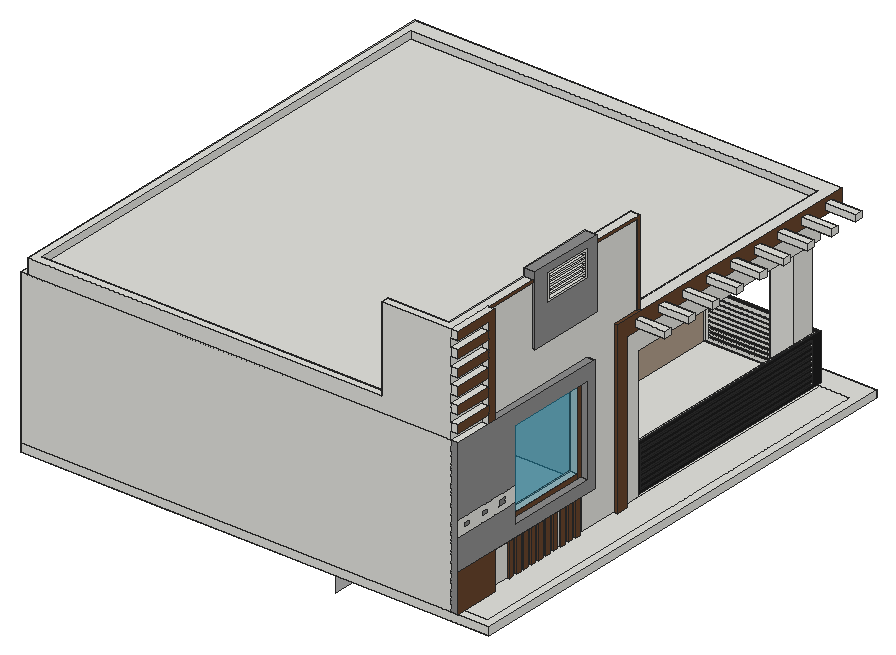
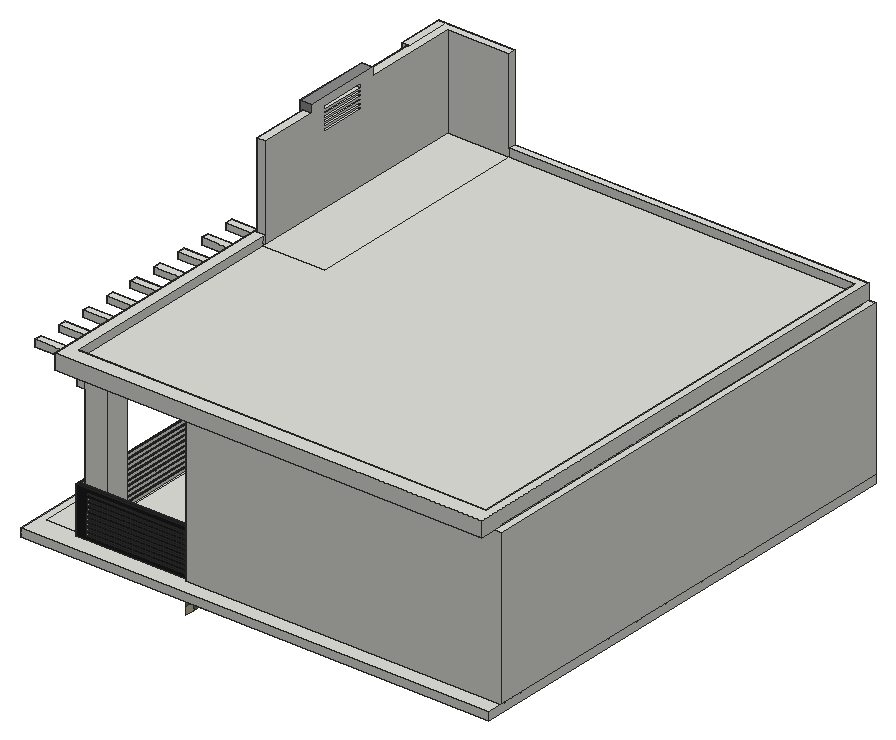
# SketchUp Ruby script. Lengths in inches.
U = 1.inch
M = Sketchup.active_model
def pt(a) = Geom::Point3d.new(a.map { |v| v * U })
def face(e, loops, mat)
  f = e.add_face(loops[0].map { |a| pt(a) })
  loops[1..].each { |l| e.add_face(l.map { |a| pt(a) }).erase! }
  f.material = f.back_material = mat if mat
  f
end
# faces: each face lists its corners as indices into pts; further lists are holes
def faces(e, pts, list, mat = nil) = list.each { |f| face(e, (f[0].is_a?(Array) ? f : [f]).map { |l| l.map { |i| pts[i] } }, mat) }
# xy, xz, yz: faces in a plane at the given z, y or x. An outline is a flat list of corners, or four numbers for a rectangle; further outlines are holes
def ring(l) = l.size == 4 ? [[l[0], l[1]], [l[2], l[1]], [l[2], l[3]], [l[0], l[3]]] : l.each_slice(2).to_a
def flat(e, list, mat, &to3) = list.each { |f| face(e, (f[0].is_a?(Array) ? f : [f]).map { |l| ring(l).map { |u, v| to3.(u, v) } }, mat) }
def xy(e, z, list, mat = nil) = flat(e, list, mat) { |x, y| [x, y, z] }
def xz(e, y, list, mat = nil) = flat(e, list, mat) { |x, z| [x, y, z] }
def yz(e, x, list, mat = nil) = flat(e, list, mat) { |y, z| [x, y, z] }
def lines(e, pts, list) = list.each { |a, b| e.add_line(pt(pts[a]), pt(pts[b])) }
# prism: a flat outline (further loops are holes) pulled along v
def prism(e, loops, v, mat = nil)
  f = face(e, loops, mat); d = Geom::Vector3d.new(v.map { |x| x * U })
  f.pushpull(f.normal.samedirection?(d) ? d.length : -d.length)
end
def box(e, o, s, mat = nil) = prism(e, [[o, [o[0] + s[0], o[1], o[2]], [o[0] + s[0], o[1] + s[1], o[2]], [o[0], o[1] + s[1], o[2]]]], [0, 0, s[2]], mat)
def at(x, y, z, deg = 0) = Geom::Transformation.translation(pt([x, y, z])) * Geom::Transformation.rotation(ORIGIN, Z_AXIS, deg.degrees)
def axes(o, x, y, z) = Geom::Transformation.new([*x, 0, *y, 0, *z, 0, *pt(o).to_a, 1])
def part(name) = M.definitions.add(name)
# library, detail: a bought-in or finely detailed component or shape, given as its bounding box
def library(name, o, s) = part(name).tap { |d| box(d.entities, o, s) }
def detail(e, o, s) = box(e.add_group.entities, o, s)
def put(e, d, t, mat = nil) = e.add_instance(d, t).tap { |i| i.material = mat if mat }
def group(e, t, mat = nil) = e.add_group.tap { |g| g.transformation = t; g.material = mat if mat }.entities
root = M.entities
M.materials.add("Brick_01_1K").color = [147, 115, 98]
M.materials.add("Brick_05_1K").color = [195, 185, 161]
M.materials.add("Brick_20_1K1").color = [126, 109, 93]
M.materials.add("Glass_Basic_01").color = [33, 150, 186]
M.materials["Glass_Basic_01"].alpha = 0.4
M.materials.add("M02_Ash_Whisper").color = [196, 196, 196]
M.materials.add("M04_Stone_Frost").color = [142, 142, 142]
M.materials.add("M08_Obsidian_Black").color = [30, 30, 30]
M.materials.add("ThomThom - Complexion2").color = [175, 156, 137]
M.materials.add("ThomThom - Waistcoat2").color = [127, 127, 126]
M.materials.add("Wood_Veneer_15_1K").color = [103, 69, 45]
xy(root,144,[[57,57,174,66],[174,57,180,66],[180,57,294,66],[294,57,303,423],[[303,57,423,435],[309,63,417,429]],
  [[309,63,309,429,417,429,417,81,405,81,405,63],[369,399,387,417]],[57,66,66,423],[66,66,174,234],[174,66,180,414],[180,66,294,234],
  [66,234,174,240],[180,234,294,240],[66,240,174,414],[180,240,294,414],[66,414,174,423],
  [174,414,180,423],[180,414,294,423],[57,423,66,435],[66,423,174,435],[174,423,180,435],
  [180,423,294,435],[294,423,303,435]])
xy(root,150,[[399,57,423,57,423,435,57,435,57,423,303,423,303,420.78,391,420.78,391,417,417,417,417,63,399,63],[63,63,174,234],[180,63,387,234],[399,63,417,63,417,417,393,417,393,225,396,225,396,216,393,216,393,180.2,395,180.2,395,176.6,393,176.6,393,173,395,173,395,169.4,393,169.4,393,165.8,395,165.8,395,162.2,393,162.2,393,158.6,395,158.6,395,155,393,155,393,151.4,395,151.4,395,147.8,393,147.8,393,144.2,395,144.2,395,140.6,393,140.6,393,137,395,137,395,133.4,393,133.4,393,129.8,395,129.8,395,126.2,393,126.2,393,122.6,395,122.6,395,119,393,119,393,115.4,395,115.4,395,111.8,393,111.8,393,93,399,93],[63,240,174,417],
  [180,240,297,417],[303,240,387,240,387,399,369,399,369,417,303,417],[387,240,393,240,393,417,391,417,391,242,389,242,389,417,387,417],[303,417,389,417.78]])
xy(root,152,[[389,244,391,413]],"M08_Obsidian_Black")
xy(root,153,[[297,255,303,297]])
xy(root,153,[[306,417.78,382.19,420.78]],"M08_Obsidian_Black")
xy(root,153.88,[[389,244,391,413]],"M08_Obsidian_Black")
xy(root,154.76,[[306,417.78,382.19,420.78]])
xy(root,155.76,[[389,244,391,413]],"M08_Obsidian_Black")
xy(root,156.53,[[306,417.78,382.19,420.78]],"M08_Obsidian_Black")
xy(root,157.65,[[389,244,391,413]],"M08_Obsidian_Black")
xy(root,158.29,[[306,417.78,382.19,420.78]],"M08_Obsidian_Black")
xy(root,159.53,[[389,244,391,413]],"M08_Obsidian_Black")
xy(root,160.06,[[306,417.78,382.19,420.78]],"M08_Obsidian_Black")
xy(root,161.41,[[389,244,391,413]],"M08_Obsidian_Black")
xy(root,161.82,[[306,417.78,382.19,420.78]],"M08_Obsidian_Black")
xy(root,163.29,[[389,244,391,413]],"M08_Obsidian_Black")
xy(root,163.59,[[306,417.78,382.19,420.78]],"M08_Obsidian_Black")
xy(root,165.18,[[389,244,391,413]],"M08_Obsidian_Black")
xy(root,165.35,[[306,417.78,382.19,420.78]],"M08_Obsidian_Black")
xy(root,167.06,[[389,244,391,413]],"M08_Obsidian_Black")
xy(root,167.12,[[306,417.78,382.19,420.78]],"M08_Obsidian_Black")
xy(root,168.88,[[306,417.78,382.19,420.78]],"M08_Obsidian_Black")
xy(root,168.94,[[389,244,391,413]],"M08_Obsidian_Black")
xy(root,170.65,[[306,417.78,382,420.78]],"M08_Obsidian_Black")
xy(root,170.82,[[389,244,391,413]],"M08_Obsidian_Black")
xy(root,172.41,[[306,417.78,382,420.78]],"M08_Obsidian_Black")
xy(root,172.71,[[389,244,391,413]],"M08_Obsidian_Black")
xy(root,174.18,[[306,417.78,382,420.78]],"M08_Obsidian_Black")
xy(root,174.59,[[389,244,391,413]],"M08_Obsidian_Black")
xy(root,175.94,[[306,417.78,382,420.78]],"M08_Obsidian_Black")
xy(root,176.47,[[389,244,391,413]],"M08_Obsidian_Black")
xy(root,177.71,[[306,417.78,382,420.78]],"M08_Obsidian_Black")
xy(root,178.35,[[389,244,391,413]],"M08_Obsidian_Black")
xy(root,179.47,[[306,417.78,382,420.78]],"M08_Obsidian_Black")
xy(root,180,[[393,93,399,111.8],[395,111.8,395,115.4,393,115.4,393,119,395,119,395,122.6,393,122.6,393,126.2,395,126.2,395,129.8,393,129.8,393,133.4,395,133.4,395,137,393,137,393,140.6,395,140.6,395,144.2,393,144.2,393,147.8,395,147.8,395,151.4,393,151.4,393,155,395,155,395,158.6,393,158.6,393,162.2,395,162.2,395,165.8,393,165.8,393,169.4,395,169.4,395,173,393,173,393,176.6,395,176.6,395,180.2,393,180.2,393,183.8,399,183.8,399,111.8],[393,183.8,399,189.8]])
xy(root,180.24,[[389,244,391,413]],"M08_Obsidian_Black")
xy(root,181.24,[[306,417.78,382,420.78]],"M08_Obsidian_Black")
xy(root,182.12,[[389,244,391,413]],"M08_Obsidian_Black")
xy(root,183,[[306,417.78,382,420.78]],"M08_Obsidian_Black")
xy(root,184,[[389,244,391,413]],"M08_Obsidian_Black")
xy(root,186,[[389,242,391,242,391,420.78,303,420.78,303,417.78,389,417.78]],"M08_Obsidian_Black")
xy(root,189,[[297,327,303,369]])
xy(root,189,[[393,111.8,399,183.8]],"M04_Stone_Frost")
xy(root,192,[[387,114.8,393,180.8]])
xy(root,231,[[297,255,303,297],[297,327,303,369]])
xy(root,252,[[381,240,381,399,387,399,387,417,393,417,393,240]])
xy(root,255,[[387,114.8,393,180.8]])
xy(root,258,[[393,111.8,399,183.8]],"M04_Stone_Frost")
xy(root,270,[[57,57,63,423],[63,57,174,63],[174,57,180,63],[180,57,387,63],[393,57,399,87],
  [63,63,174,234],[174,63,180,417],[180,63,387,234],[393,225,396,240],[63,234,174,240],
  [180,234,387,234,387,240,303,240,303,417,297,417,297,240,180,240],[393,240,393,417,303,417,303,423,63,423,63,435,396,435,396,240],[63,240,174,417],[180,240,297,417],[303,240,303,417,369,417,369,399,381,399,381,240],
  [63,417,174,423],[174,417,180,423],[180,417,297,423],[297,417,303,423]])
xy(root,270,[[393,93,399,189.8]],"M04_Stone_Frost")
xy(root,273.58,[[396,232.62,420,238.62],[396,255.85,420,261.85],[396,279.07,420,285.07],[396,302.29,420,308.29],[396,325.52,420,331.52],
  [396,348.74,420,354.74],[396,371.97,420,377.97],[396,395.19,420,401.19],[396,418.41,420,424.41]])
xy(root,276,[[69,63,339,63,339,243,387,243,387,423,69,423],[339,63,387,243]])
xy(root,276.55,[[393,57,399,87]])
xy(root,278.58,[[396,232.62,420,238.62],[396,255.85,420,261.85],[396,279.07,420,285.07],[396,302.29,420,308.29],[396,325.52,420,331.52],
  [396,348.74,420,354.74],[396,371.97,420,377.97],[396,395.19,420,401.19],[396,418.41,420,424.41]])
xy(root,282,[[63,57,339,57,339,63,69,63,69,423,387,423,387,240,396,240,396,435,63,435]])
xy(root,282,[[393,216,396,216,396,240,394,240,394,238,393,238]],"Wood_Veneer_15_1K")
xy(root,283.09,[[393,57,399,87]])
xy(root,289.64,[[393,57,399,87]])
xy(root,296.18,[[393,57,399,87]])
xy(root,300,[[393,135.8,396,195.8]])
xy(root,302.73,[[393,57,399,87]])
xy(root,309.27,[[393,57,399,87]])
xy(root,315.82,[[393,57,399,87]])
xy(root,322.36,[[393,57,399,87]])
xy(root,328.91,[[393,57,399,87]])
xy(root,329,[[396,146.8,397,184.8]])
xy(root,330,[[387,147.8,397,183.8]])
xy(root,332,[[387,147.8,396,183.8]])
xy(root,333,[[387,147.8,396,183.8]])
xy(root,335,[[387,147.8,396,183.8]])
xy(root,335.45,[[393,57,399,87]])
xy(root,336,[[387,147.8,396,183.8]])
xy(root,338,[[387,147.8,396,183.8]])
xy(root,339,[[387,147.8,396,183.8]])
xy(root,341,[[387,147.8,396,183.8]])
xy(root,342,[[393,57,399,87],[387,147.8,396,183.8]])
xy(root,344,[[387,147.8,396,183.8]])
xy(root,345,[[387,147.8,396,183.8]])
xy(root,346,[[393,93,394,135.8],[393,195.8,394,238]])
xy(root,348,[[339,57,393,57,393,93,394,93,394,135.8,387,135.8,387,63,339,63],[393,57,399,93],[387,147.8,397,183.8],[387,195.8,394,240]])
xy(root,349,[[396,146.8,397,184.8]])
xy(root,354,[[387,135.8,396,195.8]],"M04_Stone_Frost")
xz(root,57,[[57,144,423,150],[57,150,393,270],[63,270,393,270,393,348,339,348,339,282,63,282],[393,276.55,399,283.09],[393,289.64,399,296.18],
  [393,302.73,399,309.27],[393,315.82,399,322.36],[393,328.91,399,335.45],[393,342,399,348]])
xz(root,57,[[393,150,399,270]],"M04_Stone_Frost")
xz(root,63,[[63,150,174,270],[174,150,180,270],[180,150,387,270],[69,276,339,282],[339,276,387,348]])
xz(root,87,[[393,270,399,276.55],[393,283.09,399,289.64],[393,296.18,399,302.73],[393,309.27,399,315.82],[393,322.36,399,328.91],
  [393,335.45,399,342]])
xz(root,93,[[393,270,393,346,394,346,394,348,399,348,399,270]])
xz(root,93,[[393,150,399,180]],"Wood_Veneer_15_1K")
xz(root,111.8,[[393,189,399,258]],"M04_Stone_Frost")
xz(root,111.8,[[393,150,395,180]],"Wood_Veneer_15_1K")
xz(root,114.8,[[387,192,393,255]])
xz(root,115.4,[[393,150,395,180]],"Wood_Veneer_15_1K")
xz(root,119,[[393,150,395,180]],"Wood_Veneer_15_1K")
xz(root,122.6,[[393,150,395,180]],"Wood_Veneer_15_1K")
xz(root,126.2,[[393,150,395,180]],"Wood_Veneer_15_1K")
xz(root,129.8,[[393,150,395,180]],"Wood_Veneer_15_1K")
xz(root,133.4,[[393,150,395,180]],"Wood_Veneer_15_1K")
xz(root,135.8,[[393,300,396,300,396,354,387,354,387,348,394,348,394,346,393,346]],"M04_Stone_Frost")
xz(root,137,[[393,150,395,180]],"Wood_Veneer_15_1K")
xz(root,140.6,[[393,150,395,180]],"Wood_Veneer_15_1K")
xz(root,144.2,[[393,150,395,180]],"Wood_Veneer_15_1K")
xz(root,146.8,[[396,329,397,349]])
xz(root,147.8,[[387,330,397,332],[396,332,397,333],[387,333,397,335],[396,335,397,336],[387,336,397,338],
  [396,338,397,339],[387,339,397,341],[396,341,397,342],[387,342,397,344],[396,344,397,345],
  [387,345,397,348]])
xz(root,147.8,[[393,150,395,180]],"Wood_Veneer_15_1K")
xz(root,151.4,[[393,150,395,180]],"Wood_Veneer_15_1K")
xz(root,155,[[393,150,395,180]],"Wood_Veneer_15_1K")
xz(root,158.6,[[393,150,395,180]],"Wood_Veneer_15_1K")
xz(root,162.2,[[393,150,395,180]],"Wood_Veneer_15_1K")
xz(root,165.8,[[393,150,395,180]],"Wood_Veneer_15_1K")
xz(root,169.4,[[393,150,395,180]],"Wood_Veneer_15_1K")
xz(root,173,[[393,150,395,180]],"Wood_Veneer_15_1K")
xz(root,176.6,[[393,150,395,180]],"Wood_Veneer_15_1K")
xz(root,180.2,[[393,150,395,180]],"Wood_Veneer_15_1K")
xz(root,180.8,[[387,192,393,255]])
xz(root,183.8,[[387,330,397,332],[396,332,397,333],[387,333,397,335],[396,335,397,336],[387,336,397,338],
  [396,338,397,339],[387,339,397,341],[396,341,397,342],[387,342,397,344],[396,344,397,345],
  [387,345,397,348]])
xz(root,183.8,[[393,189,399,258]],"M04_Stone_Frost")
xz(root,184.8,[[396,329,397,348],[396,348,397,349]])
xz(root,189.8,[[393,180,399,186],[393,186,399,234],[393,234,399,270]],"M04_Stone_Frost")
xz(root,195.8,[[393,300,393,346,394,346,394,348,387,348,387,354,396,354,396,300]],"M04_Stone_Frost")
xz(root,216,[[393,150,396,282]],"Wood_Veneer_15_1K")
xz(root,225,[[393,150,396,270]])
xz(root,232.62,[[396,273.58,420,278.58]])
xz(root,234,[[63,150,174,270],[180,150,387,270]])
xz(root,238,[[393,282,394,346]])
xz(root,238.62,[[396,273.58,420,278.58]])
xz(root,240,[[63,150,174,270],[180,150,297,270],[303,150,381,270],[381,150,387,252],[387,150,393,252],
  [387,282,394,348]])
xz(root,242,[[389,150,391,186]])
xz(root,244,[[389,152,391,153.88],[389,155.76,391,157.65],[389,159.53,391,161.41],[389,163.29,391,165.18],[389,167.06,391,168.94],
  [389,170.82,391,172.71],[389,174.59,391,176.47],[389,178.35,391,180.24],[389,182.12,391,184]])
xz(root,255,[[297,153,303,231]])
xz(root,255.85,[[396,273.58,420,278.58]])
xz(root,261.85,[[396,273.58,420,278.58]])
xz(root,279.07,[[396,273.58,420,278.58]])
xz(root,285.07,[[396,273.58,420,278.58]])
xz(root,297,[[297,153,303,231]])
xz(root,302.29,[[396,273.58,420,278.58]])
xz(root,308.29,[[396,273.58,420,278.58]])
xz(root,325.52,[[396,273.58,420,278.58]])
xz(root,327,[[297,189,303,231]])
xz(root,331.52,[[396,273.58,420,278.58]])
xz(root,348.74,[[396,273.58,420,278.58]])
xz(root,354.74,[[396,273.58,420,278.58]])
xz(root,369,[[297,189,303,231]])
xz(root,371.97,[[396,273.58,420,278.58]])
xz(root,377.97,[[396,273.58,420,278.58]])
xz(root,395.19,[[396,273.58,420,278.58]])
xz(root,399,[[369,150,387,150,387,252,381,252,381,270,369,270]])
xz(root,401.19,[[396,273.58,420,278.58]])
xz(root,413,[[389,152,391,153.88],[389,155.76,391,157.65],[389,159.53,391,161.41],[389,163.29,391,165.18],[389,167.06,391,168.94],
  [389,170.82,391,172.71],[389,174.59,391,176.47],[389,178.35,391,180.24],[389,182.12,391,184]])
xz(root,417,[[63,150,174,270],[174,150,180,270],[180,150,297,270],[297,150,303,270],[369,150,387,270],
  [387,252,393,270]])
xz(root,417.78,[[[303,150,389,186],[306,167.12,382.19,168.88],[306,163.59,382.19,165.35],[306,160.06,382.19,161.82],[306,156.53,382.19,158.29],[306,153,382.19,154.76],[306,181.24,382,183],[306,177.71,382,179.47],[306,174.18,382,175.94],[306,170.65,382,172.41]]])
xz(root,418.41,[[396,273.58,420,278.58]])
xz(root,420.78,[[[303,150,391,186],[306,153,382.19,153,382.19,154.76,306,154.76,306,156.53,382.19,156.53,382.19,158.29,306,158.29,306,160.06,382.19,160.06,382.19,161.82,306,161.82,306,163.59,382.19,163.59,382.19,165.35,306,165.35,306,167.12,382.19,167.12,382.19,168.88,306,168.88,306,170.65,382,170.65,382,172.41,306,172.41,306,174.18,382,174.18,382,175.94,306,175.94,306,177.71,382,177.71,382,179.47,306,179.47,306,181.24,382,181.24,382,183,306,183]]],"M08_Obsidian_Black")
xz(root,423,[[57,150,303,270],[69,276,387,282]])
xz(root,424.41,[[396,273.58,420,278.58]])
xz(root,435,[[57,144,423,150],[63,270,396,282]])
yz(root,57,[[57,144,435,150],[57,150,423,270]])
yz(root,63,[[63,150,234,270],[234,150,240,270],[240,150,417,270],[57,270,435,282]])
yz(root,69,[[63,276,423,282]])
yz(root,174,[[63,150,234,270],[240,150,417,270]])
yz(root,180,[[63,150,234,270],[240,150,417,270]])
yz(root,297,[[[240,150,417,270],[255,153,297,231],[327,189,369,231]]])
yz(root,303,[[417,150,417.78,150,417.78,186,420.78,186,420.78,150,423,150,423,270,417,270]])
yz(root,303,[[253.33,132,260,138]],"Brick_01_1K")
yz(root,303,[[240,126,247.5,132],[262.5,126,270,132],[285,126,292.5,132],[307.24,126,314.47,132],[328.94,126,336.18,132],
  [350.65,126,357.88,132],[372.35,126,379.59,132],[394.06,126,401.29,132],[415.76,126,423,132],[246.67,132,253.33,138],
  [260,132,266.67,138],[280,132,286.67,138],[300,132,310.25,138],[330.75,132,341,138],[361.5,132,371.75,138],
  [392.25,132,402.5,138],[240,138,247.5,144],[255,138,262.5,144],[270,138,277.5,144],[285,138,292.5,144],
  [300,138,307.24,144],[314.47,138,321.71,144],[328.94,138,336.18,144],[343.41,138,350.65,144],[357.88,138,365.12,144],
  [372.35,138,379.59,144],[386.82,138,394.06,144],[401.29,138,408.53,144],[415.76,138,423,144]],"Brick_05_1K")
yz(root,303,[[247.5,126,255,132],[255,126,262.5,132],[270,126,277.5,132],[277.5,126,285,132],[292.5,126,300,132],
  [300,126,307.24,132],[314.47,126,321.71,132],[321.71,126,328.94,132],[336.18,126,343.41,132],[343.41,126,350.65,132],
  [357.88,126,365.12,132],[365.12,126,372.35,132],[379.59,126,386.82,132],[386.82,126,394.06,132],[401.29,126,408.53,132],
  [408.53,126,415.76,132],[240,132,246.67,138],[266.67,132,273.33,138],[273.33,132,280,138],[286.67,132,293.33,138],
  [293.33,132,300,138],[310.25,132,320.5,138],[320.5,132,330.75,138],[341,132,351.25,138],[351.25,132,361.5,138],
  [371.75,132,382,138],[382,132,392.25,138],[402.5,132,412.75,138],[412.75,132,423,138],[247.5,138,255,144],
  [262.5,138,270,144],[277.5,138,285,144],[292.5,138,300,144],[307.24,138,314.47,144],[321.71,138,328.94,144],
  [336.18,138,343.41,144],[350.65,138,357.88,144],[365.12,138,372.35,144],[379.59,138,386.82,144],[394.06,138,401.29,144],
  [408.53,138,415.76,144]],"Brick_20_1K1")
yz(root,303,[[327,189,369,231]],"Glass_Basic_01")
yz(root,303,[[57,132,222,144]],"M02_Ash_Whisper")
yz(root,303,[[[240,150,252,150,252,234,300,234,300,150,417,150,417,270,240,270],[324,186,372,234]]],"ThomThom - Complexion2")
yz(root,303,[[[252,150,300,234],[255,153,297,231]],[[324,186,372,234],[327,189,369,231]]],"Wood_Veneer_15_1K")
yz(root,306,[[417.78,153,420.78,154.76],[417.78,156.53,420.78,158.29],[417.78,160.06,420.78,161.82],[417.78,163.59,420.78,165.35],[417.78,167.12,420.78,168.88],
  [417.78,170.65,420.78,172.41],[417.78,174.18,420.78,175.94],[417.78,177.71,420.78,179.47],[417.78,181.24,420.78,183]])
yz(root,339,[[57,282,63,348]])
yz(root,369,[[399,150,417,270]])
yz(root,381,[[240,252,399,270]])
yz(root,382,[[417.78,170.65,420.78,172.41],[417.78,174.18,420.78,175.94],[417.78,177.71,420.78,179.47],[417.78,181.24,420.78,183]])
yz(root,382.19,[[417.78,153,420.78,154.76],[417.78,156.53,420.78,158.29],[417.78,160.06,420.78,161.82],[417.78,163.59,420.78,165.35],[417.78,167.12,420.78,168.88]])
yz(root,387,[[[63,150,234,270],[114.8,192,180.8,255]],[399,150,417,252],[[63,276,63,348,135.8,348,135.8,354,195.8,354,195.8,348,240,348,240,276],[147.8,345,183.8,348],[147.8,342,183.8,344],[147.8,339,183.8,341],[147.8,336,183.8,338],[147.8,333,183.8,335],[147.8,330,183.8,332]],[240,276,243,282],[243,276,423,282]])
yz(root,387,[[114.8,192,180.8,255]],"Glass_Basic_01")
yz(root,389,[[242,150,242,186,399,186,399,184,244,184,244,182.12,399,182.12,399,180.24,244,180.24,244,178.35,399,178.35,399,176.47,244,176.47,244,174.59,399,174.59,399,172.71,244,172.71,244,170.82,399,170.82,399,168.94,244,168.94,244,167.06,399,167.06,399,165.18,244,165.18,244,163.29,399,163.29,399,161.41,244,161.41,244,159.53,399,159.53,399,157.65,244,157.65,244,155.76,399,155.76,399,153.88,244,153.88,244,152,399,152,399,150],[399,150,399,152,413,152,413,153.88,399,153.88,399,155.76,413,155.76,413,157.65,399,157.65,399,159.53,413,159.53,413,161.41,399,161.41,399,163.29,413,163.29,413,165.18,399,165.18,399,167.06,413,167.06,413,168.94,399,168.94,399,170.82,413,170.82,413,172.71,399,172.71,399,174.59,413,174.59,413,176.47,399,176.47,399,178.35,413,178.35,413,180.24,399,180.24,399,182.12,413,182.12,413,184,399,184,399,186,417.78,186,417.78,150],[399,152,413,153.88],[399,155.76,413,157.65],[399,159.53,413,161.41],
  [399,163.29,413,165.18],[399,167.06,413,168.94],[399,170.82,413,172.71],[399,174.59,413,176.47],[399,178.35,413,180.24],
  [399,182.12,413,184]])
yz(root,391,[[[242,150,420.78,186],[244,152,413,184]],[244,153.88,413,155.76],[244,157.65,413,159.53],[244,161.41,413,163.29],[244,165.18,413,167.06],
  [244,168.94,413,170.82],[244,172.71,413,174.59],[244,176.47,413,178.35],[244,180.24,413,182.12]],"M08_Obsidian_Black")
yz(root,393,[[183.8,150,216,150,216,282,238,282,238,346,195.8,346,195.8,300,135.8,300,135.8,346,93,346,93,270,189.8,270,189.8,180,183.8,180],[93,150,111.8,180],[115.4,150,119,180],[122.6,150,126.2,180],[129.8,150,133.4,180],
  [137,150,140.6,180],[144.2,150,147.8,180],[151.4,150,155,180],[158.6,150,162.2,180],[165.8,150,169.4,180],
  [173,150,176.6,180],[180.2,150,183.8,180],[225,150,240,150,240,252,417,252,417,270,225,270],[57,270,87,276.55],[57,283.09,87,289.64],
  [57,296.18,87,302.73],[57,309.27,87,315.82],[57,322.36,87,328.91],[57,335.45,87,342]])
yz(root,393,[[114.8,192,180.8,255]],"Glass_Basic_01")
yz(root,393,[[111.8,189,114.8,189,114.8,255,180.8,255,180.8,189,183.8,189,183.8,258,111.8,258],[114.8,189,180.8,192]],"Wood_Veneer_15_1K")
yz(root,394,[[238,282,240,282,240,348,195.8,348,195.8,346,238,346],[93,346,135.8,348]],"Wood_Veneer_15_1K")
yz(root,395,[[111.8,150,115.4,180],[119,150,122.6,180],[126.2,150,129.8,180],[133.4,150,137,180],[140.6,150,144.2,180],
  [147.8,150,151.4,180],[155,150,158.6,180],[162.2,150,165.8,180],[169.4,150,173,180],[176.6,150,180.2,180]],"Wood_Veneer_15_1K")
yz(root,396,[[147.8,332,183.8,333],[147.8,335,183.8,336],[147.8,338,183.8,339],[147.8,341,183.8,342],[147.8,344,183.8,345]])
yz(root,396,[[[135.8,300,195.8,354],[146.8,329,184.8,349]]],"M04_Stone_Frost")
yz(root,396,[[[216,150,225,150,225,270,435,270,435,282,216,282],[232.62,273.58,238.62,278.58],[279.07,273.58,285.07,278.58],[302.29,273.58,308.29,278.58],[325.52,273.58,331.52,278.58],[348.74,273.58,354.74,278.58],[371.97,273.58,377.97,278.58],[395.19,273.58,401.19,278.58],[418.41,273.58,424.41,278.58],[255.85,273.58,261.85,278.58]]],"Wood_Veneer_15_1K")
yz(root,397,[[[146.8,329,184.8,349],[147.8,330,183.8,348]]])
yz(root,399,[[[57,204,111.8,216],[80.2,208.37,86.2,212.37],[62.03,208.37,68.03,212.37],[96.73,208.37,102.73,212.37]]])
yz(root,399,[[57,180,189.8,180,189.8,270,57,270,57,216,111.8,216,111.8,258,183.8,258,183.8,189,111.8,189,111.8,204,57,204]],"M04_Stone_Frost")
yz(root,399,[[62.03,208.37,68.03,212.37],[80.2,208.37,86.2,212.37],[96.73,208.37,102.73,212.37]],"ThomThom - Waistcoat2")
yz(root,399,[[57,150,93,180],[87,270,93,270,93,348,57,348,57,342,87,342],[57,276.55,87,283.09],[57,289.64,87,296.18],[57,302.73,87,309.27],
  [57,315.82,87,322.36],[57,328.91,87,335.45]],"Wood_Veneer_15_1K")
yz(root,420,[[232.62,273.58,238.62,278.58],[255.85,273.58,261.85,278.58],[279.07,273.58,285.07,278.58],[302.29,273.58,308.29,278.58],[325.52,273.58,331.52,278.58],
  [348.74,273.58,354.74,278.58],[371.97,273.58,377.97,278.58],[395.19,273.58,401.19,278.58],[418.41,273.58,424.41,278.58]])
yz(root,423,[[57,144,435,150]])
p = [[387,240,270],[393,240,270],[387,417,150],[387,417,144]]
lines(root,p,[[0,1],[2,3]])
